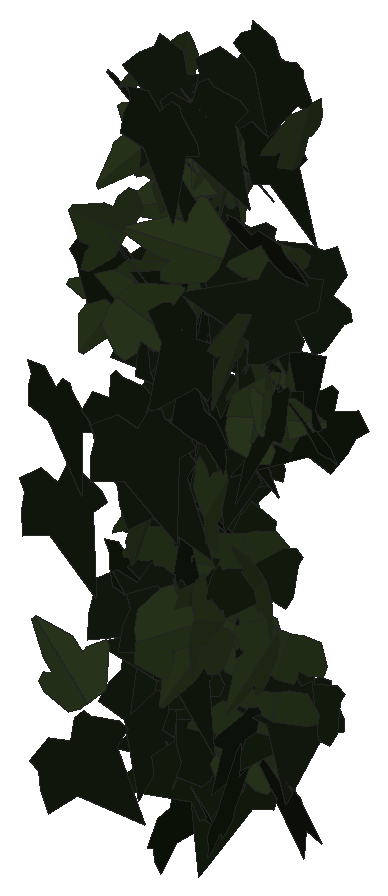
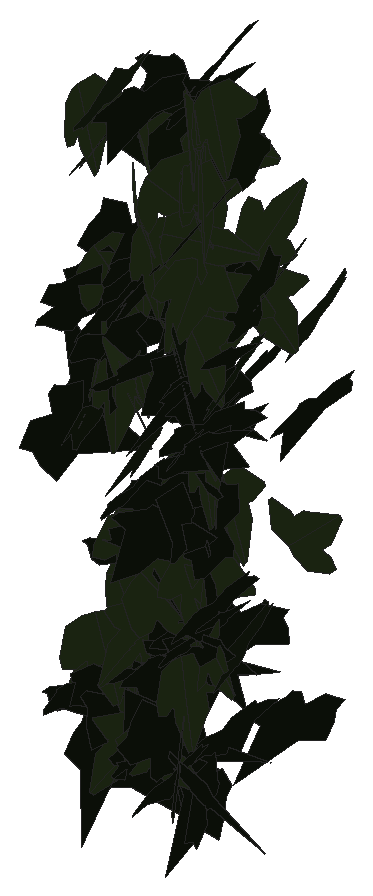
# SketchUp Ruby script. Lengths in inches.
U = 1.inch
M = Sketchup.active_model
def pt(a) = Geom::Point3d.new(a.map { |v| v * U })
def face(e, loops, mat)
  f = e.add_face(loops[0].map { |a| pt(a) })
  loops[1..].each { |l| e.add_face(l.map { |a| pt(a) }).erase! }
  f.material = f.back_material = mat if mat
  f
end
# faces: each face lists its corners as indices into pts; further lists are holes
def faces(e, pts, list, mat = nil) = list.each { |f| face(e, (f[0].is_a?(Array) ? f : [f]).map { |l| l.map { |i| pts[i] } }, mat) }
# xy, xz, yz: faces in a plane at the given z, y or x. An outline is a flat list of corners, or four numbers for a rectangle; further outlines are holes
def ring(l) = l.size == 4 ? [[l[0], l[1]], [l[2], l[1]], [l[2], l[3]], [l[0], l[3]]] : l.each_slice(2).to_a
def flat(e, list, mat, &to3) = list.each { |f| face(e, (f[0].is_a?(Array) ? f : [f]).map { |l| ring(l).map { |u, v| to3.(u, v) } }, mat) }
def xy(e, z, list, mat = nil) = flat(e, list, mat) { |x, y| [x, y, z] }
def xz(e, y, list, mat = nil) = flat(e, list, mat) { |x, z| [x, y, z] }
def yz(e, x, list, mat = nil) = flat(e, list, mat) { |y, z| [x, y, z] }
def lines(e, pts, list) = list.each { |a, b| e.add_line(pt(pts[a]), pt(pts[b])) }
# prism: a flat outline (further loops are holes) pulled along v
def prism(e, loops, v, mat = nil)
  f = face(e, loops, mat); d = Geom::Vector3d.new(v.map { |x| x * U })
  f.pushpull(f.normal.samedirection?(d) ? d.length : -d.length)
end
def box(e, o, s, mat = nil) = prism(e, [[o, [o[0] + s[0], o[1], o[2]], [o[0] + s[0], o[1] + s[1], o[2]], [o[0], o[1] + s[1], o[2]]]], [0, 0, s[2]], mat)
def at(x, y, z, deg = 0) = Geom::Transformation.translation(pt([x, y, z])) * Geom::Transformation.rotation(ORIGIN, Z_AXIS, deg.degrees)
def axes(o, x, y, z) = Geom::Transformation.new([*x, 0, *y, 0, *z, 0, *pt(o).to_a, 1])
def part(name) = M.definitions.add(name)
# library, detail: a bought-in or finely detailed component or shape, given as its bounding box
def library(name, o, s) = part(name).tap { |d| box(d.entities, o, s) }
def detail(e, o, s) = box(e.add_group.entities, o, s)
def put(e, d, t, mat = nil) = e.add_instance(d, t).tap { |i| i.material = mat if mat }
def group(e, t, mat = nil) = e.add_group.tap { |g| g.transformation = t; g.material = mat if mat }.entities
root = M.entities
M.materials.add("efeu1").color = [18, 25, 13]
M.materials.add("efeu2").color = [43, 57, 29]
c1 = part("ivyleaf_10")
p = [[0,0.5,-0.03],[-0.0625,2.02,-0.43],[-0.19,2.01,-0.46],[-0.54,1.05,-0.29],[-0.52,0.625,-0.18],[-0.83,0.76,-0.28],
  [-1.16,0.64,-0.33],[-1.15,0.33,-0.24],[-0.77,-0.39,0.02],[-0.3,-0.51,0.16],[0.04,-0.48,0.23],[-0.02,2.01,-0.4375],
  [-0.06,2.01,-0.43],[0.04,-0.49,0.23],[0.67,-0.49,0.14],[1.38,0.36,-0.2],[1.375,0.51,-0.24],[0.81,0.65,-0.19],
  [0.62,0.59,-0.15],[0.6,1.09,-0.28],[0.5,1.23,-0.31]]
faces(c1.entities,p,[[0,1,2,3,4,5,6,7,8,9,10],[11,12,0,13,14,15,16,17,18,19,20]],"efeu2")
c2 = part("ivyleaf_9")
p = [[1.54,2.16,1.25],[1.36,2.04,1.19],[-0.21,0.99,0.68],[-0.71,1.11,0.82],[-0.85,0.86,0.67],[-0.8,0.17,0.21],
  [-0.9,-0.01,0.1],[-0.67,-0.16,-0.02],[-0.08,-0.08,-0.05],[-0.03,-0.6,-0.4],[0.65,-0.88,-0.66],[0.83,-0.6,-0.49],
  [1.29,-0.42,-0.43],[1.8125,-0.07,-0.26],[1.21,0.44,0.15]]
faces(c2.entities,p,[[0,1,2,3,4,5,6,7,8,9,10,11,12,13,14]],"efeu1")
put(root,c1,axes([28.62,219.75,225.59],[0.34622,0.08558,0.35044],[-0.34366,-0.06943,0.35648],[0.10967,-0.48771,0.01075]))
put(root,c2,axes([27.94,220.15,229.41],[0.19409,-0.4425,0.12855],[0.04367,-0.1212,-0.48312],[0.45872,0.19876,-0.0084]))
put(root,c2,axes([29.4,219.97,229.39],[-0.19712,-0.23869,-0.39265],[0.26348,0.29133,-0.30937],[0.37646,-0.32887,0.01092]))
put(root,c2,axes([28.03,220.09,228.08],[0.12781,-0.45468,-0.16411],[-0.02696,0.16278,-0.47199],[0.48264,0.12949,0.0171]))
put(root,c2,axes([28.9,221.04,233.33],[0.11221,-0.48082,0.07884],[0.01798,-0.07676,-0.49374],[0.48691,0.11365,0.00006]))
put(root,c2,axes([27.66,220.84,223.91],[0.09324,-0.27229,-0.40886],[-0.02838,0.41248,-0.28117],[0.49041,0.07564,0.06147]))
put(root,c2,axes([28.23,220.92,229.02],[0.2763,-0.32759,-0.25757],[-0.09636,0.25044,-0.42189],[0.40543,0.28278,0.07526]))
put(root,c1,axes([29.72,220.75,226.48],[0.1126,-0.22856,-0.43021],[-0.01878,0.43919,-0.23825],[0.48679,0.06981,0.09032]))
put(root,c2,axes([29.07,221.49,229.95],[-0.0563,-0.36956,0.33205],[-0.06935,-0.32506,-0.37353],[0.49196,-0.08812,-0.01465]))
put(root,c1,axes([27.85,221.49,231.125],[-0.10764,-0.27417,-0.40404],[-0.16124,-0.37057,0.29442],[-0.46088,0.19368,-0.00864]))
put(root,c1,axes([28.93,220.83,225.95],[0.01554,-0.02579,-0.49909],[0.27761,0.41565,-0.01283],[0.41556,-0.27671,0.02724]))
put(root,c2,axes([29.16,221.5625,228.93],[0.32157,-0.27676,-0.26457],[0.19985,-0.17338,0.42426],[-0.32658,-0.37861,-0.00089]))
put(root,c1,axes([29.25,221.45,231.32],[0.10813,0.14194,0.46708],[-0.30483,-0.35403,0.17816],[0.3813,-0.32329,0.00997]))
put(root,c1,axes([28.02,221.41,230.3],[-0.27321,-0.31412,0.27691],[-0.15495,-0.23133,-0.4153],[0.38903,-0.31275,0.02906]))
put(root,c1,axes([28.4375,221.06,230.34],[0.24673,0.19842,0.38698],[0.2054,0.339,-0.30478],[-0.38332,0.30937,0.08578]))
put(root,c2,axes([28.52,221.27,228.03],[0.20367,-0.36434,-0.27528],[-0.04008,0.28599,-0.40817],[0.45488,0.18833,0.08729]))
put(root,c1,axes([29.16,221.64,225.59],[-0.13021,-0.37674,0.30185],[-0.05839,-0.29805,-0.39719],[0.4792,-0.13868,0.03362]))
put(root,c2,axes([29.875,221.05,223.42],[0.07659,0.12608,0.47774],[-0.05857,0.48236,-0.11791],[-0.49061,-0.0379,0.08866]))
put(root,c1,axes([28.28,221.77,232.55],[-0.10258,-0.18885,0.45146],[-0.03538,-0.4572,-0.19929],[0.48808,-0.07283,0.08044]))
put(root,c2,axes([27.57,221.44,230.73],[0.30326,-0.36624,-0.15459],[-0.07261,0.14013,-0.47444],[0.39084,0.31021,0.03181]))
put(root,c1,axes([29.86,221.93,225.59],[-0.00603,-0.21839,0.44974],[0.15997,-0.42697,-0.20519],[0.47368,0.14142,0.07502]))
put(root,c2,axes([28.99,221.6,233.23],[-0.11063,-0.18953,-0.44927],[0.35749,0.28177,-0.2069],[0.3316,-0.367,0.07316]))
put(root,c1,axes([28.21,221.68,227.31],[0.07064,-0.4933,0.04075],[0.01105,-0.03958,-0.49831],[0.49486,0.0713,0.00531]))
put(root,c1,axes([29.5,221.88,230.05],[0.11347,-0.42613,0.23567],[0.08176,-0.22188,-0.44055],[0.48004,0.13851,0.01933]))
put(root,c2,axes([28.49,222.03,233.3],[-0.14893,-0.43383,0.19902],[-0.02322,-0.20165,-0.45694],[0.47674,-0.14535,0.03992]))
put(root,c1,axes([28.74,221.76,226],[0.03091,-0.49844,0.02462],[0.00221,-0.02453,-0.49939],[0.49904,0.03098,0.00068]))
put(root,c2,axes([27.61,221.85,230.58],[0.31269,-0.29163,0.25919],[0.18431,-0.18235,-0.42753],[0.34388,0.36291,-0.00653]))
put(root,c2,axes([28.58,221.85,225.2],[0.21027,-0.45356,-0.00813],[-0.00229,0.0079,-0.49993],[0.45363,0.21028,0.00124]))
put(root,c2,axes([27.67,221.8125,232.97],[0.46952,-0.17146,0.01242],[0.01139,-0.00503,-0.49984],[0.17153,0.46966,-0.00082]))
put(root,c1,axes([28.18,221.85,230.4375],[-0.42951,-0.25594,-0.00343],[0.00313,0.00146,-0.49999],[0.25595,-0.42953,0.00035]))
put(root,c1,axes([29.23,221.55,227.55],[0.10795,0.00185,-0.4882],[-0.07471,0.49417,-0.01465],[0.48246,0.07612,0.10697]))
put(root,c1,axes([28.71,222.27,230.47],[-0.00181,-0.29632,0.40273],[0.14797,-0.38501,-0.28261],[0.4776,0.11816,0.08909]))
put(root,c2,axes([27.8125,221.96,225.74],[-0.10724,-0.3535,-0.33695],[0.12775,0.31266,-0.36868],[0.47136,-0.16516,0.02325]))
put(root,c2,axes([28.95,222.19,223.51],[-0.40042,-0.04721,0.29569],[-0.27904,-0.12026,-0.39708],[0.10861,-0.48302,0.06996]))
put(root,c2,axes([27.85,222.26,224.125],[-0.05445,-0.49158,0.07335],[-0.00802,-0.07291,-0.49459],[0.49696,-0.05504,0.00005]))
put(root,c1,axes([28.81,221.98,232.57],[-0.4767,0.06696,-0.13518],[0.1331,-0.02424,-0.48135],[-0.07102,-0.4949,0.00528]))
put(root,c1,axes([28.34,222.1,232.3125],[-0.00407,-0.49994,-0.0066],[0.00008,0.0066,-0.49996],[0.49998,-0.00407,0.00002]))
put(root,c2,axes([28.71,222.16,232.71],[0.35128,-0.27139,0.23011],[0.18062,-0.14259,-0.4439],[0.30656,0.39499,-0.00214]))
put(root,c2,axes([28.65,222.36,229.85],[0.00078,0.05485,0.49698],[-0.38313,-0.31926,0.03583],[0.32126,-0.38088,0.04153]))
put(root,c1,axes([28.3125,222.17,232.2],[-0.02641,-0.49515,0.06427],[-0.00514,-0.06408,-0.49585],[0.49928,-0.02685,-0.00171]))
put(root,c1,axes([29.16,222.23,232.43],[0.2673,-0.40696,0.11373],[0.06684,-0.09215,-0.48687],[0.41723,0.27549,0.00514]))
put(root,c2,axes([29.81,222.23,229.07],[-0.40332,0.09303,-0.28049],[0.27436,-0.05847,-0.4139],[-0.10981,-0.48778,-0.00388]))
put(root,c2,axes([28.52,221.76,222.89],[-0.00321,-0.01327,-0.49981],[-0.33393,0.37206,-0.00774],[0.37213,0.33375,-0.01125]))
put(root,c2,axes([28.22,222.19,225.5],[-0.0933,-0.42615,-0.24432],[0.08125,0.23187,-0.43547],[0.48445,-0.12096,0.02598]))
put(root,c1,axes([28.07,222.17,233.42],[-0.0478,-0.49731,0.02005],[0.00168,-0.02031,-0.49958],[0.49771,-0.04769,0.00361]))
put(root,c1,axes([28.28,222.12,228.09],[0.05367,-0.49313,-0.06278],[-0.00455,0.06265,-0.49604],[0.49709,0.05382,0.00224]))
put(root,c2,axes([28.72,222.25,224.86],[-0.3083,0.08778,0.38372],[-0.39326,-0.04756,-0.30509],[-0.01706,-0.48993,0.09837]))
put(root,c2,axes([28.72,221.74,230.32],[-0.07322,0.16844,-0.46504],[-0.35276,0.31173,0.16846],[0.34669,0.35277,0.07319]))
put(root,c1,axes([28.24,222.1,228.1],[0.38801,-0.315,0.01497],[-0.00199,0.02128,0.49954],[-0.31535,-0.38771,0.01526]))
put(root,c2,axes([28.13,222.33,222.99],[0.28821,-0.07325,-0.40196],[0.40281,-0.03141,0.29455],[-0.0684,-0.49361,0.0409]))
put(root,c1,axes([29.33,222.21,224.3125],[-0.32706,-0.37162,0.07021],[-0.04082,-0.05759,-0.49499],[0.37599,-0.32951,0.00733]))
put(root,c2,axes([29.9,222.41,230.16],[-0.20032,0.01375,0.45791],[-0.43324,-0.16813,-0.18448],[0.1489,-0.47069,0.07928]))
put(root,c2,axes([28.06,222.36,226.53],[0.03903,-0.0935,-0.48963],[0.49847,0.00879,0.03806],[0.00149,-0.4911,0.0939]))
put(root,c1,axes([29.73,221.97,226.45],[0.30303,-0.08426,-0.38868],[-0.24285,0.34777,-0.26472],[0.31495,0.34922,0.16984]))
put(root,c2,axes([28.59,222.42,228.97],[-0.45143,-0.135,0.1673],[-0.1616,-0.04351,-0.47116],[0.14177,-0.47946,-0.00435]))
put(root,c2,axes([28.19,222.375,225.35],[-0.46002,-0.14246,-0.1345],[0.12817,0.04081,-0.48157],[0.14819,-0.47754,-0.00103]))
put(root,c1,axes([28.41,222.44,231.39],[-0.08624,-0.02086,0.49206],[-0.32692,-0.3712,-0.07303],[0.36836,-0.33433,0.05039]))
put(root,c2,axes([27.96,222.21,227.12],[0.40305,-0.13139,0.26511],[0.2472,-0.09668,-0.42373],[0.16261,0.47264,-0.01297]))
put(root,c2,axes([29.65,222.29,232.68],[0.26763,-0.41486,-0.07915],[-0.02748,0.0764,-0.49336],[0.42145,0.26843,0.01809]))
put(root,c2,axes([29.49,222.36,224.23],[-0.07742,0.33242,-0.36538],[0.07968,-0.35659,-0.34131],[-0.4875,-0.11108,0.00223]))
put(root,c2,axes([28.89,222.5,223.33],[-0.29685,-0.39452,-0.07894],[0.04962,0.06145,-0.49372],[0.39927,-0.30096,0.00267]))
put(root,c2,axes([27.33,222.4375,225.68],[0.25492,-0.42189,0.0838],[0.03272,-0.07811,-0.49278],[0.42889,0.25672,-0.01221]))
put(root,c2,axes([29.01,222.57,231],[-0.17037,-0.46821,0.04186],[-0.01525,-0.039,-0.49824],[0.46983,-0.17104,-0.001]))
put(root,c1,axes([28.17,222.29,226.43],[-0.3724,-0.33143,-0.03841],[0.02866,0.02557,-0.49852],[0.33242,-0.3735,-0.00005]))
put(root,c2,axes([29.4,222.6,226.57],[-0.43776,-0.23473,0.05717],[-0.05305,-0.02203,-0.49669],[0.2357,-0.44093,-0.00562]))
put(root,c1,axes([29.25,222.33,226.6875],[-0.37823,-0.32661,-0.01639],[0.01209,0.01108,-0.49973],[0.3268,-0.37842,-0.00049]))
put(root,c2,axes([28.57,222.43,224.98],[-0.03357,-0.45022,-0.21488],[0.04061,0.21219,-0.45092],[0.49722,-0.04773,0.02232]))
put(root,c1,axes([29.66,222.39,224.51],[-0.37538,-0.32691,0.04715],[-0.03353,-0.0333,-0.49776],[0.32859,-0.37686,0.00308]))
put(root,c1,axes([29.59,222.2,229.14],[0.15454,-0.1706,-0.44386],[-0.3202,0.30771,-0.22975],[0.35155,0.35526,-0.01415]))
put(root,c1,axes([29.5,222.06,228.72],[0.03058,0.07897,0.49278],[0.19795,0.45129,-0.0846],[-0.45813,0.20026,-0.00366]))
put(root,c2,axes([27.99,222.73,225.68],[-0.1103,-0.45878,0.1654],[0.0137,-0.17243,-0.46913],[0.48749,-0.09896,0.05061]))
put(root,c2,axes([28.96,222.2,223.46],[-0.24562,-0.15626,0.40651],[0.32895,0.2393,0.29074],[-0.28542,0.41026,-0.01475]))
put(root,c1,axes([28.37,222.33,233.3],[0.30643,-0.34955,-0.18417],[-0.05049,0.19651,-0.45698],[0.39186,0.29866,0.08514]))
put(root,c1,axes([29.56,222.63,230.75],[-0.15124,-0.40285,0.25464],[-0.04617,-0.25351,-0.42849],[0.47434,-0.15313,0.03948]))
put(root,c2,axes([28.29,222.51,229.7],[-0.05002,0.31024,0.38891],[0.05577,-0.38491,0.31422],[0.49436,0.07482,0.0039]))
put(root,c2,axes([28.56,222.38,225.01],[-0.39856,0.08776,0.28887],[0.24352,-0.18934,0.39351],[0.17846,0.45436,0.10819]))
put(root,c1,axes([28.17,222.29,225.39],[-0.16017,0.0264,0.47292],[-0.45969,0.11165,-0.16192],[-0.11415,-0.48666,-0.01149]))
put(root,c2,axes([27.375,222.56,229.83],[0.26705,-0.42254,-0.01206],[-0.00643,0.01021,-0.49985],[0.42266,0.26713,0.00002]))
put(root,c1,axes([29.98,222.54,232.96],[0.01425,-0.4985,0.03602],[0.01532,-0.03558,-0.4985],[0.49956,0.01531,0.01425]))
put(root,c2,axes([27.95,222.74,231.86],[0.09251,-0.47403,0.12936],[0.02927,-0.12608,-0.48296],[0.49049,0.09693,0.00442]))
put(root,c2,axes([28.59,222.62,227.68],[-0.22325,-0.40451,-0.19112],[0.08222,0.17286,-0.46191],[0.43977,-0.23767,-0.01067]))
put(root,c2,axes([29.38,222.32,231.17],[0.40316,0.12861,-0.2663],[-0.26006,-0.06021,-0.42278],[-0.14081,0.47941,0.01834]))
put(root,c2,axes([27.82,222.67,228.875],[0.12706,-0.4835,0.00894],[0.00243,-0.00861,-0.49992],[0.48358,0.12708,0.00016]))
put(root,c2,axes([28.74,222.47,230.86],[0.24158,-0.38083,-0.21589],[-0.06159,0.21456,-0.4474],[0.43341,0.24276,0.05676]))
put(root,c2,axes([29.77,222.38,223.38],[0.39227,0.01304,-0.30977],[-0.30882,-0.02784,-0.39224],[-0.02748,0.49905,-0.01379]))
put(root,c2,axes([28.97,222.54,233.4375],[0.03443,-0.42926,-0.25406],[-0.00578,0.25431,-0.43046],[0.49878,0.03258,0.01255]))
put(root,c1,axes([28.68,222.7,226.16],[-0.26135,-0.24146,0.35128],[-0.2566,-0.2399,-0.35581],[0.34037,-0.36626,0.00148]))
put(root,c1,axes([28.2,222.41,230.86],[-0.24463,-0.38299,-0.20851],[0.11601,0.1733,-0.45443],[0.42035,-0.27071,0.00407]))
put(root,c2,axes([28.47,222.22,228.8125],[-0.0099,0.10546,0.48865],[-0.1163,0.47485,-0.10484],[-0.48619,-0.11574,0.01513]))
put(root,c2,axes([28.1,222.5,229.53],[0.16145,0.37405,-0.28986],[-0.13712,-0.25616,-0.40692],[-0.45292,0.21088,0.01987]))
put(root,c1,axes([28.46,222.9,232.39],[-0.08669,-0.32716,0.36803],[0.13885,-0.37477,-0.30044],[0.47245,0.05011,0.15583]))
put(root,c2,axes([27.72,222.91,229.87],[-0.13873,-0.46884,0.1046],[0.0214,-0.1148,-0.48617],[0.47989,-0.13041,0.05192]))
put(root,c1,axes([29.28,222.8,229.92],[0.18126,-0.421,0.19976],[0.06506,-0.18938,-0.45815],[0.46143,0.19208,-0.01387]))
put(root,c1,axes([28.21,222.63,224.97],[-0.10194,-0.4894,-0.00986],[0.00242,0.00957,-0.4999],[0.48949,-0.10197,0.00042]))
put(root,c2,axes([28.69,222.58,228.53],[0.33952,-0.34139,-0.13483],[-0.08932,0.10129,-0.48142],[0.35602,0.35099,0.00779]))
put(root,c2,axes([29.29,222.97,233.39],[-0.02803,-0.402,0.29599],[0.09552,-0.2953,-0.39202],[0.48999,0.03457,0.09335]))
put(root,c2,axes([27.72,222.82,229],[-0.13469,-0.47514,-0.0781],[0.01565,0.07674,-0.49383],[0.48126,-0.13547,-0.0058]))
put(root,c2,axes([28.4,222.29,227.15],[-0.01771,-0.05198,0.49698],[0.13736,0.47762,0.05485],[-0.48044,0.13847,-0.00264]))
put(root,c1,axes([29.76,222.34,228.6],[0.03352,0.39898,-0.29948],[-0.04285,0.30135,0.39668],[0.49703,-0.00093,0.0544]))
put(root,c1,axes([28.84,222.7,223.8125],[0.33375,0.01429,-0.37203],[-0.37097,-0.02958,-0.33393],[-0.03156,0.49892,-0.00914]))
put(root,c2,axes([27.88,222.98,228.6],[-0.27095,-0.39147,0.15278],[-0.0573,-0.14567,-0.47487],[0.4163,-0.27484,0.03408]))
put(root,c1,axes([29.6,222.71,225.19],[-0.3863,-0.27966,0.1502],[-0.10754,-0.1073,-0.47636],[0.29867,-0.40034,0.02276]))
put(root,c2,axes([29.67,222.89,224.49],[-0.11132,-0.48708,-0.01896],[0.00537,0.01823,-0.49964],[0.48742,-0.11144,0.00117]))
put(root,c2,axes([28.49,222.94,223.84],[0.04667,0.03587,0.49652],[-0.39315,-0.30326,0.05886],[0.30538,-0.39591,-0.0001]))
put(root,c1,axes([29.13,222.4,223.66],[0.21157,0.29973,0.3397],[0.11956,0.32469,-0.36095],[-0.43697,0.23396,0.06572]))
put(root,c2,axes([28.47,222.625,227.12],[-0.08365,-0.25196,-0.4237],[0.24636,0.35087,-0.25729],[0.42698,-0.25181,0.06545]))
put(root,c2,axes([28.2,222.95,223.59],[0.03754,-0.49285,0.07542],[0.01194,-0.07473,-0.49424],[0.49845,0.03891,0.00616]))
put(root,c2,axes([28.72,223.04,227.84],[-0.07035,-0.47181,0.14983],[0.00675,-0.15224,-0.47621],[0.49498,-0.06498,0.02779]))
put(root,c2,axes([29.71,223.04,224.5],[-0.35141,-0.33392,0.12252],[-0.08346,-0.09,-0.4847],[0.34575,-0.36111,0.00752]))
put(root,c2,axes([29.54,222.89,228.78],[-0.10131,0.05092,0.48697],[0.26041,-0.41552,0.09762],[0.41464,0.2734,0.05768]))
put(root,c1,axes([28.69,222.74,231.4],[-0.00298,-0.49629,-0.06072],[-0.01682,0.06079,-0.49601],[0.49971,-0.00091,-0.01705]))
put(root,c1,axes([27.71,222.92,230.24],[0.08332,-0.46287,0.16972],[0.05311,-0.16269,-0.4698],[0.49014,0.09632,0.02205]))
put(root,c2,axes([27.48,222.93,226.45],[0.05558,-0.4962,-0.02639],[-0.00599,0.02588,-0.49929],[0.49687,0.05581,-0.00307]))
put(root,c2,axes([28.1,222.74,223.54],[-0.42609,0.19136,0.17839],[-0.15728,0.08508,-0.46693],[-0.20906,-0.45403,-0.01231]))
put(root,c1,axes([28.99,222.4375,225.41],[0.08318,0.29886,0.39213],[-0.00312,0.39798,-0.30266],[-0.49302,0.04791,0.06808]))
put(root,c2,axes([29.93,223.13,230.18],[-0.26086,-0.19536,0.37919],[-0.27897,-0.25811,-0.32489],[0.32269,-0.38107,0.02566]))
put(root,c1,axes([28.67,223.01,231.98],[0.27155,-0.17652,0.38093],[0.31294,-0.21732,-0.32379],[0.27987,0.41426,-0.00754]))
put(root,c2,axes([29.75,223.03,228.34],[0.29349,-0.40093,0.05588],[-0.03028,0.04709,0.49686],[-0.40367,-0.29502,0.00336]))
put(root,c2,axes([27.95,223.1,223.86],[0.0758,-0.123,-0.47867],[0.44887,-0.1855,0.11875],[-0.2068,-0.44773,0.0823]))
put(root,c1,axes([27.78,222.74,232.6],[0.17166,-0.44532,-0.14908],[0.0011,0.15911,-0.47401],[0.46961,0.16241,0.05561]))
put(root,c2,axes([29.98,223.11,228.49],[-0.10666,0.02949,-0.4876],[0.00971,-0.49886,-0.03229],[-0.48839,-0.01636,0.10585]))
put(root,c2,axes([29.09,222.95,230.47],[0.09289,-0.48571,-0.07387],[-0.02622,0.07017,-0.49436],[0.4906,0.09571,-0.01244]))
put(root,c2,axes([27.97,222.62,229.54],[0.2543,-0.25292,-0.34837],[-0.10595,0.35539,-0.33537],[0.41726,0.24439,0.12716]))
put(root,c1,axes([29.24,222.76,229.22],[-0.0477,-0.47806,-0.13852],[-0.00413,0.13953,-0.48012],[0.4977,-0.04466,-0.01726]))
put(root,c2,axes([29.13,223.09,230.01],[-0.22811,-0.44488,0.00717],[-0.00331,-0.00636,-0.49995],[0.44492,-0.22813,-0.00005]))
put(root,c2,axes([28.82,223.22,229.59],[-0.24655,-0.36381,0.23844],[-0.03953,-0.25421,-0.42874],[0.43319,-0.23026,0.09659]))
